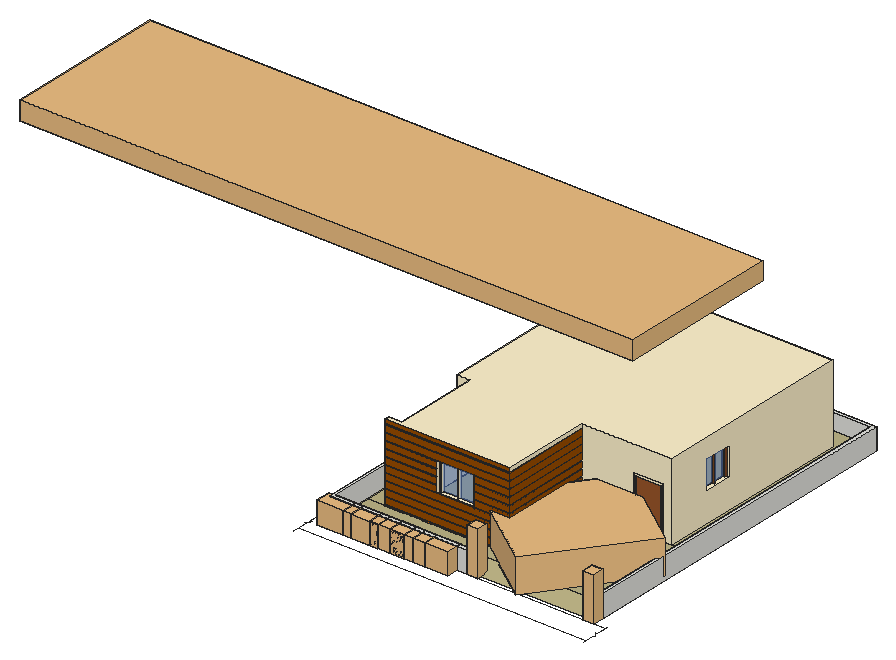
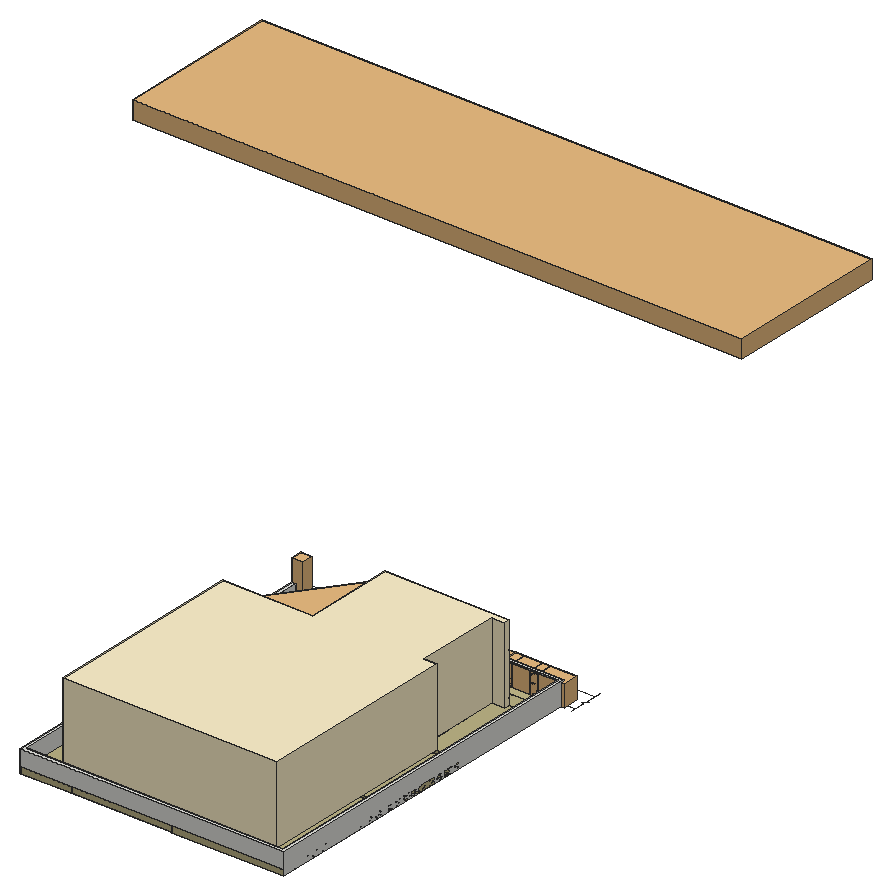
# SketchUp Ruby script. Lengths in inches.
U = 1.inch
M = Sketchup.active_model
def pt(a) = Geom::Point3d.new(a.map { |v| v * U })
def face(e, loops, mat)
  f = e.add_face(loops[0].map { |a| pt(a) })
  loops[1..].each { |l| e.add_face(l.map { |a| pt(a) }).erase! }
  f.material = f.back_material = mat if mat
  f
end
# faces: each face lists its corners as indices into pts; further lists are holes
def faces(e, pts, list, mat = nil) = list.each { |f| face(e, (f[0].is_a?(Array) ? f : [f]).map { |l| l.map { |i| pts[i] } }, mat) }
# xy, xz, yz: faces in a plane at the given z, y or x. An outline is a flat list of corners, or four numbers for a rectangle; further outlines are holes
def ring(l) = l.size == 4 ? [[l[0], l[1]], [l[2], l[1]], [l[2], l[3]], [l[0], l[3]]] : l.each_slice(2).to_a
def flat(e, list, mat, &to3) = list.each { |f| face(e, (f[0].is_a?(Array) ? f : [f]).map { |l| ring(l).map { |u, v| to3.(u, v) } }, mat) }
def xy(e, z, list, mat = nil) = flat(e, list, mat) { |x, y| [x, y, z] }
def xz(e, y, list, mat = nil) = flat(e, list, mat) { |x, z| [x, y, z] }
def yz(e, x, list, mat = nil) = flat(e, list, mat) { |y, z| [x, y, z] }
def lines(e, pts, list) = list.each { |a, b| e.add_line(pt(pts[a]), pt(pts[b])) }
# prism: a flat outline (further loops are holes) pulled along v
def prism(e, loops, v, mat = nil)
  f = face(e, loops, mat); d = Geom::Vector3d.new(v.map { |x| x * U })
  f.pushpull(f.normal.samedirection?(d) ? d.length : -d.length)
end
def box(e, o, s, mat = nil) = prism(e, [[o, [o[0] + s[0], o[1], o[2]], [o[0] + s[0], o[1] + s[1], o[2]], [o[0], o[1] + s[1], o[2]]]], [0, 0, s[2]], mat)
def at(x, y, z, deg = 0) = Geom::Transformation.translation(pt([x, y, z])) * Geom::Transformation.rotation(ORIGIN, Z_AXIS, deg.degrees)
def axes(o, x, y, z) = Geom::Transformation.new([*x, 0, *y, 0, *z, 0, *pt(o).to_a, 1])
def part(name) = M.definitions.add(name)
# library, detail: a bought-in or finely detailed component or shape, given as its bounding box
def library(name, o, s) = part(name).tap { |d| box(d.entities, o, s) }
def detail(e, o, s) = box(e.add_group.entities, o, s)
def put(e, d, t, mat = nil) = e.add_instance(d, t).tap { |i| i.material = mat if mat }
def group(e, t, mat = nil) = e.add_group.tap { |g| g.transformation = t; g.material = mat if mat }.entities
root = M.entities
M.materials.add("[Color C06]").color = [204, 102, 0]
M.materials.add("[Color C07]").color = [153, 76, 0]
M.materials.add("[Color C08]").color = [102, 51, 0]
M.materials.add("[Color D01]").color = [255, 242, 204]
M.materials.add("[Color M06]").color = [86, 86, 86]
M.materials.add("[Tile Ceramic Natural]").color = [189, 180, 134]
M.materials.add("[Translucent Glass Blue]").color = [100, 149, 237]
M.materials["[Translucent Glass Blue]"].alpha = 0.5
M.materials.add("[Wood Cherry Original]").color = [152, 86, 42]
M.materials.add("[Wood Veneer 01]").color = [120, 70, 37]
c1 = library("lvt__Defintion3",[-70.01,-133.44,604.33],[1000,265.15,30.32])
c2 = library("Group\#14",[0,0,0],[56.8,25.91,35.15])
c3 = library("Group\#15",[0,0,0],[56.8,25.91,35.15])
c4 = part("House+plant_11")
put(c4.entities,c1,at(96.28,168.2,0))
put(c4.entities,c2,at(305.6,289.78,0))
put(c4.entities,c2,at(349.27,289.78,0))
put(c4.entities,c3,at(392.14,289.78,0))
put(c4.entities,c2,at(425.32,289.78,0))
put(c4.entities,c2,at(463.51,289.78,0))
c5 = library("Group172\#1",[8097.16,1237.06,0],[18,18,72])
c6 = library("002 Bmw M4 + mat3.4 2017",[-252.8,19.48,9.01],[196.94,171.32,55.15])
c7 = part("new bloSDFck")
p = [[-0.99,-2.25,0],[-22.01,-2.25,0],[-0.99,-4.5,0],[-0.99,0,0],[0.99,0,0],[0.99,-4.5,0],
  [-24,-4.5,0],[-24,0,0],[-22.01,0,0],[-22.01,-4.5,0],[22.01,-4.5,0],[22.01,0,0],
  [24,0,0],[24,-4.5,0],[24,4.5,0],[-24,4.5,0],[22.01,-2.25,0],[0.99,-2.25,0]]
lines(c7.entities,p,[[0,1],[2,3],[4,5],[6,7],[7,8],[8,9],[10,11],[11,12],[12,13],[13,6],[13,14],[6,15],
  [15,14],[12,7],[16,17]])
c8 = part("A$C63CB6BFC")
p = [[-24,-4.5,0],[24,-4.5,0],[24,0,0],[-24,0,0],[22.01,2.25,0],[1.02,2.25,0],
  [-0.96,2.25,0],[-22.01,2.25,0],[-0.96,4.5,0],[-0.96,0,0],[1.02,0,0],[1.02,4.5,0],
  [-22.01,0,0],[-22.01,4.5,0],[22.01,0,0],[24,4.5,0],[-24,4.5,0],[22.01,4.5,0]]
lines(c8.entities,p,[[0,1],[2,3],[4,5],[6,7],[8,9],[9,10],[10,11],[3,12],[12,13],[14,2],[15,16],[15,1],
  [16,0],[17,14]])
c9 = part("A$C1F62275E")
p = [[30,-4.5,0],[-30,-4.5,0],[-30,0,0],[30,0,0],[-28.01,2.25,0],[-0.99,2.25,0],
  [0.99,2.25,0],[28.01,2.25,0],[0.99,4.5,0],[0.99,0,0],[-0.99,0,0],[-0.99,4.5,0],
  [28.01,0,0],[28.01,4.5,0],[-28.01,4.5,0],[-28.01,0,0],[-30,4.5,0],[30,4.5,0]]
lines(c9.entities,p,[[0,1],[2,3],[4,5],[6,7],[8,9],[9,10],[10,11],[3,12],[12,13],[14,15],[15,2],[16,17],
  [16,1],[17,0]])
c10 = part("VEN")
p = [[-4.5,-11.98,0],[4.5,-11.98,0],[2.25,10,0],[2.25,-10,0],[0,-11.98,0],[0,11.98,0],
  [0,-10,0],[4.5,-10,0],[4.5,10,0],[0,10,0],[4.5,11.98,0],[-4.5,11.98,0]]
lines(c10.entities,p,[[0,1],[2,3],[4,5],[6,7],[8,9],[1,10],[0,11],[10,11]])
c11 = part("Group92\#2")
xy(c11.entities,0,[[0,0,25,44]],"[Translucent Glass Blue]")
c12 = part("Group90\#1")
xy(c12.entities,0,[[0,0,0,48,60,48,60,0,56,0,56,44,31,44,31,0,29,0,29,44,4,44,4,0]])
xy(c12.entities,4,[[0,0,4,0,4,44,29,44,29,0,31,0,31,44,56,44,56,0,60,0,60,48,0,48]],"[Color M06]")
xz(c12.entities,0,[[0,0,4,4],[29,0,31,4],[56,0,60,4]])
xz(c12.entities,44,[[4,0,29,4],[31,0,56,4]])
xz(c12.entities,48,[[0,0,60,4]])
yz(c12.entities,0,[[0,0,48,4]])
yz(c12.entities,4,[[0,0,44,4]])
yz(c12.entities,29,[[0,0,44,4]])
yz(c12.entities,31,[[0,0,44,4]])
yz(c12.entities,56,[[0,0,44,4]])
yz(c12.entities,60,[[0,0,48,4]])
p = [[29,0,0],[4,0,0],[56,0,0],[31,0,0],[0.08,0.08,0],[0.08,0.08,4]]
lines(c12.entities,p,[[0,1],[2,3],[4,5]])
put(c12.entities,c11,at(4,0,2))
put(c12.entities,c11,at(31,0,2))
c13 = part("Group103\#2")
xy(c13.entities,0,[[0,0,19,44]],"[Translucent Glass Blue]")
c14 = part("Group101\#1")
prism(c14.entities,[[[25,44,0],[25,0,0],[23,0,0],[23,44,0],[4,44,0],[4,0,0],[0,0,0],[0,48,0],[48,48,0],[48,0,0],[44,0,0],[44,44,0]]],[0,0,4],"[Wood Veneer 01]")
p = [[44,0,0],[25,0,0],[23,0,0],[4,0,0],[0.08,0.08,0],[0.08,0.08,4]]
lines(c14.entities,p,[[0,1],[2,3],[4,5]])
put(c14.entities,c13,at(4,0,2))
put(c14.entities,c13,at(25,0,2))
c15 = part("Group104\#1")
prism(c15.entities,[[[24,42,0],[24,-42,0],[20,-42,0],[20,38,0],[-20,38,0],[-20,-42,0],[-24,-42,0],[-24,42,0]]],[0,0,5.875])
xy(root,10,[[14.3125,35.45,426,35.45,426,208.5,246,208.5,246,60,14.3125,60]],"[Tile Ceramic Natural]")
xz(root,208.5,[[334,10,374,90]],"[Wood Cherry Original]")
p = [[330,208.5,94],[330,208.5,10],[378,208.5,10],[378,208.5,94],[82.3,510.4,0],[82.31,510.39,0],
  [78.09,524.73,0],[78.08,524.73,0],[82.28,510.42,0],[82.29,510.41,0],[82.43,510.33,0],[82.45,510.33,0],
  [78.04,524.72,0],[78.03,524.71,0],[78.02,524.71,0],[78.01,524.7,0],[78,524.69,0],[77.99,524.68,0],
  [78.1,524.73,0],[82.34,510.37,0],[82.35,510.36,0],[82.32,510.38,0],[82.33,510.375,0],[77.98,524.67,0],
  [77.97,524.66,0],[77.96,524.65,0],[77.95,524.64,0],[82.27,510.43,0],[82.26,510.46,0],[82.27,510.44,0],
  [82.4,510.34,0],[82.41,510.34,0],[82.37,510.35,0],[82.38,510.34,0],[82.42,510.33,0],[82.26,510.47,0],
  [78.07,524.73,0],[77.94,524.63,0],[77.9375,524.62,0],[82.36,510.35,0],[78.05,524.72,0],[77.93,524.61,0],
  [77.92,524.58,0],[77.92,524.57,0],[77.92,524.56,0],[77.93,524.6,0],[114.3,524.71,0],[114.29,524.7,0],
  [114.28,524.69,0],[114.39,524.73,0],[114.37,524.73,0],[114.35,524.73,0],[114.33,524.72,0],[114.27,524.68,0],
  [114.4,524.73,0],[114.36,524.73,0],[114.32,524.72,0],[114.31,524.71,0],[114.24,524.65,0],[114.23,524.64,0],
  [114.2,524.55,0],[114.2,524.53,0],[114.21,524.61,0],[114.21,524.6,0],[114.25,524.66,0],[114.2,524.57,0],
  [114.2,524.56,0],[114.26,524.67,0],[114.23,524.63,0],[114.22,524.62,0],[114.21,524.58,0],[55.55,524.73,0],
  [55.54,524.72,0],[55.58,524.73,0],[55.57,524.73,0],[51.83,524.66,0],[51.82,524.67,0],[51.875,524.53,0],
  [51.875,524.55,0],[51.81,524.68,0],[51.83,524.65,0],[51.87,524.58,0],[51.86,524.6,0],[51.8,524.69,0],
  [51.79,524.7,0],[51.85,524.63,0],[51.84,524.64,0],[51.87,524.57,0],[51.85,524.62,0],[51.875,524.56,0],
  [51.86,524.61,0],[102.17,511.09,0],[102.18,511.09,0],[102.12,511.12,0],[102.13,511.11,0],[102.07,511.18,0],
  [102.07,511.17,0],[102.0625,511.19,0],[102.14,511.1,0],[102.15,511.1,0],[102.1,511.14,0],[102.11,511.125,0],
  [102.19,511.08,0],[102.06,511.2,0],[102.08,511.16,0],[102.09,511.15,0]]
lines(root,p,[[0,1],[2,3],[4,5],[6,7],[8,9],[10,11],[12,13],[14,15],[15,16],[16,17],[18,6],[19,20],
  [21,22],[23,24],[25,26],[9,4],[27,8],[22,19],[28,29],[30,31],[32,33],[29,27],[34,10],[35,28],
  [31,34],[7,36],[5,21],[17,23],[24,25],[26,37],[37,38],[39,32],[36,40],[13,14],[20,39],[33,30],
  [40,12],[38,41],[42,43],[43,44],[45,42],[41,45],[46,47],[47,48],[49,50],[51,52],[48,53],[54,49],
  [50,55],[55,51],[52,56],[57,46],[56,57],[58,59],[60,61],[62,63],[64,58],[65,66],[53,67],[67,64],
  [68,69],[63,70],[59,68],[69,62],[70,65],[66,60],[71,72],[73,74],[74,71],[75,76],[77,78],[76,79],
  [80,75],[81,82],[83,84],[85,86],[87,81],[86,80],[88,85],[79,83],[78,89],[82,90],[89,87],[90,88],
  [91,92],[93,94],[95,96],[97,95],[94,98],[99,91],[100,101],[92,102],[101,93],[103,97],[104,105],[96,104],
  [105,100],[98,99]])
put(root,c4,at(-311.65,-308.5,0),"[Color C07]")
g1 = group(root,at(42,60,0),"[Tile Ceramic Natural]")
xy(g1,0,[[-27.6875,-54,-27.6875,148.5,21,148.5,21,100.5,30,100.5,30,157.5,-42,157.5,-42,301.5,9,301.5,9,306,-42,306,-42,516,141,516,141,468,306,468,306,516,389.04,516,389.04,-54],[9,148.5,21,153]])
xy(g1,1,[[141,468,306,477],[141,477,306,516]])
xy(g1,10,[[-27.6875,-24.55,389.04,-24.55,389.04,516,306,516,306,468,141,468,141,516,-42,516,-42,306,9,306,9,301.5,-42,301.5,-42,157.5,30,157.5,30,100.5,21,100.5,21,148.5,-27.6875,148.5],[21,100.5,30,153],[0,148.5,9,157.5],[9,148.5,21,153],[9,153,30,157.5],
  [0,301.5,9,306],[141,477,306,516]])
xz(g1,100.5,[[21,0,30,10]])
xz(g1,148.5,[[-27.6875,0,9,10],[9,0,21,10]])
xz(g1,153,[[9,0,21,10]])
xz(g1,157.5,[[-42,0,30,10],[9,10,30,130]])
xz(g1,301.5,[[-42,0,9,10]])
xz(g1,306,[[-42,0,9,10]])
xz(g1,468,[[141,0,145.5,1],[145.5,0,306,1],[141,1,145.5,10],[145.5,1,306,10]])
xz(g1,477,[[141,1,306,10]])
xz(g1,516,[[-42,0,141,10],[306,0,389.04,10],[141,1,306,10]])
yz(g1,-42,[[157.5,0,301.5,10],[306,0,516,10]])
yz(g1,-27.6875,[[-54,0,-24.55,10,148.5,10,148.5,0]])
yz(g1,9,[[148.5,0,153,10],[301.5,0,306,10],[301.5,10,306,130]])
yz(g1,21,[[100.5,0,148.5,10],[148.5,0,153,10]])
yz(g1,30,[[100.5,0,153,10],[153,0,157.5,10],[153,10,157.5,130]])
yz(g1,141,[[468,0,516,1],[468,1,477,10],[477,1,516,10]])
yz(g1,306,[[468,0,516,1],[468,1,477,10],[477,1,516,10]])
yz(g1,389.04,[[-54,0,516,0,516,10,-24.55,10]])
p = [[389.04,-24.55,10],[384,-24.55,10],[-27.6875,-24.55,10],[-27.6875,-54,0],[389.04,-54,0],[145.5,468,10],
  [145.5,468,130],[204,148.5,10],[384,148.5,10]]
faces(g1,p,[[0,1,2,3,4]])
lines(g1,p,[[5,6],[7,8],[8,1]])
put(root,c5,at(-7683.16,-1237.06,0))
put(root,c5,at(-7872.16,-1237.06,0))
g2 = group(root,at(-21.27,-51.32,0))
xy(g2,0,[[21.27,51.32,21.27,627.32,453.27,627.32,453.27,69.32,447.27,69.32,447.27,621.32,27.27,621.32,27.27,57.32,246.27,57.32,246.27,51.32],[435.27,51.32,453.27,51.32,453.27,65.32,447.27,65.32,447.27,69.32,435.27,69.32],[447.27,65.32,453.27,69.32]])
xy(g2,36,[[21.27,51.32,246.27,51.32,246.27,57.32,27.27,57.32,27.27,621.32,447.27,621.32,447.27,65.32,453.27,65.32,453.27,627.32,21.27,627.32]])
xz(g2,51.32,[[21.27,0,246.27,36]])
xz(g2,57.32,[[27.27,0,246.27,36]])
xz(g2,65.32,[[447.27,0,453.27,36]])
xz(g2,621.32,[[27.27,0,447.27,36]])
xz(g2,627.32,[[21.27,0,453.27,36]])
yz(g2,21.27,[[51.32,0,627.32,36]])
yz(g2,27.27,[[57.32,0,621.32,36]])
yz(g2,246.27,[[51.32,0,57.32,36]])
yz(g2,447.27,[[65.32,0,69.32,36],[69.32,0,621.32,36]])
yz(g2,453.27,[[65.32,0,627.32,36]])
p = [[3.02,34.2,0],[3.02,51.32,0],[246.27,69.32,0],[264.27,69.32,0],[471.91,51.32,0],[453.27,51.32,0],
  [471.91,26.49,0],[474.93,26.49,0],[468.5,34.2,0],[471.91,11.05,0],[3.02,11.05,0],[264.27,51.32,0],
  [435.27,51.32,0],[471.91,34.2,0],[21.27,51.32,0],[3.02,26.49,0],[0,26.49,0],[6.44,34.2,0],
  [3.02,0,0],[471.91,5.47,0],[246.27,51.32,0],[471.91,55.57,0],[3.02,60,0],[246.27,57.32,0]]
lines(g2,p,[[0,1],[2,3],[4,5],[6,7],[7,8],[9,10],[11,12],[13,4],[3,11],[14,1],[8,13],[10,15],
  [15,16],[17,0],[18,10],[19,9],[16,17],[20,11],[4,21],[1,22],[23,2],[9,6]])
put(root,c6,at(130.44,52.04,0,-126.296))
put(root,c7,at(46.5,289.5,10,90))
put(root,c8,axes([144,532.5,10],[1,0,0],[0,-1,0],[0,0,1]))
put(root,c9,at(158,64.5,10))
put(root,c10,at(214.58,532.5,10,-90))
g3 = group(root,at(-18.27,-51.32,10),"[Color D01]")
xy(g3,0,[[396.27,259.82,396.27,268.82,402.27,268.82,402.27,579.32,366.27,579.32,366.27,588.32,411.27,588.32,411.27,259.82],[364.27,579.32,366.27,584.82]])
xy(g3,0,[[60.27,111.32,264.27,113.32],[60.27,113.32,60.27,120.32,81.27,120.32,81.27,211.82,90.27,211.82,90.27,120.32,255.27,120.32,255.27,268.82,348.27,268.82,348.27,259.82,262.27,259.82,262.27,113.32],[262.27,113.32,264.27,259.82]],"[Color C06]")
xy(g3,1.9375,[[262.27,113.32,264.27,259.82]])
xy(g3,1.9375,[[60.27,111.32,262.27,113.32],[262.27,111.32,264.27,113.32]],"[Color C06]")
xy(g3,11.8125,[[60.27,111.32,262.27,113.32],[262.27,111.32,264.27,113.32],[262.27,113.32,264.27,259.82]],"[Color C06]")
xy(g3,13.75,[[60.27,111.32,262.27,113.32],[262.27,111.32,264.27,113.32],[262.27,113.32,264.27,259.82]])
xy(g3,23.625,[[60.27,111.32,262.27,113.32],[262.27,111.32,264.27,113.32],[262.27,113.32,264.27,259.82]],"[Color C06]")
xy(g3,25.5625,[[262.27,113.32,264.27,259.82]])
xy(g3,25.5625,[[60.27,111.32,262.27,113.32],[262.27,111.32,264.27,113.32]],"[Color C06]")
xy(g3,35.4375,[[60.27,111.32,262.27,113.32],[262.27,111.32,264.27,113.32],[262.27,113.32,264.27,259.82]],"[Color C06]")
xy(g3,37.375,[[60.27,111.32,262.27,113.32],[262.27,111.32,264.27,113.32],[262.27,113.32,264.27,259.82]])
xy(g3,47.25,[[262.27,113.32,264.27,259.82]],"[Color C06]")
xy(g3,47.25,[[60.27,111.32,262.27,113.32],[262.27,111.32,264.27,113.32]],"[Color C08]")
xy(g3,48,[[402.27,328.82,411.27,376.82]])
xy(g3,48.08,[[146.35,111.32,206.35,113.32],[146.35,113.32,206.35,120.32]])
xy(g3,49.1875,[[60.27,111.32,146.35,113.32],[262.27,113.32,264.27,259.82]])
xy(g3,49.1875,[[206.35,111.32,262.27,113.32],[262.27,111.32,264.27,113.32]],"[Color C06]")
xy(g3,59.0625,[[60.27,111.32,146.35,113.32]])
xy(g3,59.0625,[[262.27,113.32,264.27,259.82]],"[Color C06]")
xy(g3,59.0625,[[206.35,111.32,262.27,113.32],[262.27,111.32,264.27,113.32]],"[Color C08]")
xy(g3,61,[[60.27,111.32,146.35,113.32],[262.27,113.32,264.27,259.82]])
xy(g3,61,[[206.35,111.32,262.27,113.32],[262.27,111.32,264.27,113.32]],"[Color C06]")
xy(g3,70.875,[[60.27,111.32,146.35,113.32]])
xy(g3,70.875,[[262.27,113.32,264.27,259.82]],"[Color C06]")
xy(g3,70.875,[[206.35,111.32,262.27,113.32],[262.27,111.32,264.27,113.32]],"[Color C08]")
xy(g3,72.8125,[[60.27,111.32,146.35,113.32],[206.35,111.32,262.27,113.32],[262.27,111.32,264.27,113.32],[262.27,113.32,264.27,259.82]])
xy(g3,82.6875,[[60.27,111.32,146.35,113.32]])
xy(g3,82.6875,[[262.27,113.32,264.27,259.82]],"[Color C06]")
xy(g3,82.6875,[[206.35,111.32,262.27,113.32],[262.27,111.32,264.27,113.32]],"[Color C08]")
xy(g3,84,[[348.27,259.82,396.27,268.82]])
xy(g3,84.625,[[60.27,111.32,146.35,113.32],[206.35,111.32,262.27,113.32],[262.27,111.32,264.27,113.32],[262.27,113.32,264.27,259.82]])
xy(g3,94.5,[[60.27,111.32,146.35,113.32]])
xy(g3,94.5,[[262.27,113.32,264.27,259.82]],"[Color C06]")
xy(g3,94.5,[[206.35,111.32,262.27,113.32],[262.27,111.32,264.27,113.32]],"[Color C08]")
xy(g3,96,[[402.27,328.82,411.27,376.82]])
xy(g3,96.08,[[146.35,111.32,206.35,120.32]])
xy(g3,96.4375,[[262.27,113.32,264.27,259.82]])
xy(g3,96.4375,[[60.27,111.32,262.27,113.32],[262.27,111.32,264.27,113.32]],"[Color C06]")
xy(g3,106.3125,[[262.27,113.32,264.27,259.82]],"[Color C06]")
xy(g3,106.3125,[[60.27,111.32,262.27,113.32],[262.27,111.32,264.27,113.32]],"[Color C08]")
xy(g3,108.25,[[60.27,111.32,262.27,113.32],[262.27,111.32,264.27,113.32],[262.27,113.32,264.27,259.82]])
xy(g3,118.125,[[262.27,113.32,264.27,259.82]],"[Color C06]")
xy(g3,118.125,[[60.27,111.32,262.27,113.32],[262.27,111.32,264.27,113.32]],"[Color C08]")
xy(g3,120.0625,[[262.27,113.32,264.27,259.82]],"[Color C06]")
xy(g3,120.0625,[[60.27,111.32,262.27,113.32],[262.27,111.32,264.27,113.32]],"[Color C08]")
xy(g3,126,[[60.27,111.32,264.27,111.32,264.27,259.82,411.27,259.82,411.27,588.32,60.27,588.32,60.27,259.82,81.27,259.82,81.27,120.32,60.27,120.32]])
xz(g3,111.32,[[60.27,1.9375,264.27,11.8125],[60.27,13.75,264.27,23.625],[60.27,25.5625,264.27,35.4375],[60.27,37.375,264.27,47.25],[60.27,49.1875,146.35,59.0625],
  [206.35,49.1875,264.27,59.0625],[60.27,61,146.35,70.875],[206.35,61,264.27,70.875],[60.27,72.8125,146.35,82.6875],[206.35,72.8125,264.27,82.6875],
  [60.27,84.625,146.35,94.5],[206.35,84.625,264.27,94.5],[60.27,96.4375,264.27,106.3125],[60.27,108.25,264.27,118.125],[60.27,120.0625,264.27,126]],"[Color C07]")
xz(g3,113.32,[[60.27,0,262.27,1.9375],[262.27,0,264.27,1.9375],[60.27,11.8125,262.27,13.75],[262.27,11.8125,264.27,13.75],[60.27,23.625,262.27,25.5625],
  [262.27,23.625,264.27,25.5625],[60.27,35.4375,262.27,37.375],[262.27,35.4375,264.27,37.375],[60.27,47.25,262.27,47.25,262.27,49.1875,206.35,49.1875,206.35,48.08,146.35,48.08,146.35,49.1875,60.27,49.1875],[262.27,47.25,264.27,49.1875],
  [60.27,59.0625,146.35,61],[206.35,59.0625,262.27,61],[262.27,59.0625,264.27,61],[60.27,70.875,146.35,72.8125],[206.35,70.875,262.27,72.8125],
  [262.27,70.875,264.27,72.8125],[60.27,82.6875,146.35,84.625],[206.35,82.6875,262.27,84.625],[262.27,82.6875,264.27,84.625],[262.27,94.5,264.27,96.4375],
  [60.27,106.3125,262.27,108.25],[262.27,106.3125,264.27,108.25]],"[Color C06]")
xz(g3,113.32,[[60.27,118.125,262.27,120.0625],[262.27,118.125,264.27,120.0625]],"[Color C08]")
xz(g3,120.32,[[60.27,0,81.27,126],[[90.27,0,255.27,120],[146.35,48.08,206.35,96.08]]])
xz(g3,259.82,[[60.27,0,81.27,126]])
xz(g3,259.82,[[264.27,0,348.27,0,348.27,84,396.27,84,396.27,0,411.27,0,411.27,126,264.27,126]],"[Color D01]")
xz(g3,268.82,[[255.27,0,255.27,120,402.27,120,402.27,0,396.27,0,396.27,84,348.27,84,348.27,0]])
xz(g3,328.82,[[402.27,48,411.27,96]])
xz(g3,376.82,[[402.27,48,411.27,96]])
xz(g3,579.32,[[69.27,0,201.27,120],[205.77,0,259.77,120],[264.27,0,402.27,120]],"[Color D01]")
xz(g3,588.32,[[60.27,0,411.27,126]],"[Color D01]")
yz(g3,60.27,[[111.32,0,113.32,1.9375],[113.32,0,113.32,1.9375,111.32,1.9375,111.32,11.8125,113.32,11.8125,113.32,13.75,111.32,13.75,111.32,23.625,113.32,23.625,113.32,25.5625,111.32,25.5625,111.32,35.4375,113.32,35.4375,113.32,37.375,111.32,37.375,111.32,47.25,113.32,47.25,113.32,49.1875,111.32,49.1875,111.32,59.0625,113.32,59.0625,113.32,61,111.32,61,111.32,70.875,113.32,70.875,113.32,72.8125,111.32,72.8125,111.32,82.6875,113.32,82.6875,113.32,84.625,111.32,84.625,111.32,94.5,113.32,94.5,113.32,96.4375,111.32,96.4375,111.32,106.3125,113.32,106.3125,113.32,108.25,111.32,108.25,111.32,118.125,113.32,118.125,113.32,120.0625,111.32,120.0625,111.32,126,120.32,126,120.32,0],[259.82,0,588.32,126],[111.32,11.8125,113.32,13.75],[111.32,23.625,113.32,25.5625],
  [111.32,35.4375,113.32,37.375],[111.32,47.25,113.32,49.1875],[111.32,59.0625,113.32,61],[111.32,70.875,113.32,72.8125],[111.32,82.6875,113.32,84.625],
  [111.32,94.5,113.32,96.4375],[111.32,106.3125,113.32,108.25],[111.32,118.125,113.32,120.0625]])
yz(g3,69.27,[[268.82,0,412.82,120],[417.32,0,579.32,120]])
yz(g3,81.27,[[120.32,0,259.82,126]])
yz(g3,90.27,[[120.32,0,264.32,120]])
yz(g3,146.35,[[111.32,48.08,113.32,49.1875],[113.32,48.08,120.32,48.08,120.32,96.08,113.32,96.08,113.32,94.5,111.32,94.5,111.32,84.625,113.32,84.625,113.32,82.6875,111.32,82.6875,111.32,72.8125,113.32,72.8125,113.32,70.875,111.32,70.875,111.32,61,113.32,61,113.32,59.0625,111.32,59.0625,111.32,49.1875,113.32,49.1875],[111.32,59.0625,113.32,61],[111.32,70.875,113.32,72.8125],[111.32,82.6875,113.32,84.625],
  [111.32,94.5,113.32,96.08]])
yz(g3,206.35,[[111.32,48.08,113.32,49.1875],[113.32,48.08,113.32,49.1875,111.32,49.1875,111.32,59.0625,113.32,59.0625,113.32,61,111.32,61,111.32,70.875,113.32,70.875,113.32,72.8125,111.32,72.8125,111.32,82.6875,113.32,82.6875,113.32,84.625,111.32,84.625,111.32,94.5,113.32,94.5,113.32,96.08,120.32,96.08,120.32,48.08],[111.32,59.0625,113.32,61],[111.32,70.875,113.32,72.8125],[111.32,82.6875,113.32,84.625],
  [111.32,94.5,113.32,96.08]])
yz(g3,255.27,[[120.32,0,268.82,120]])
yz(g3,262.27,[[113.32,0,259.82,1.9375],[113.32,11.8125,259.82,13.75],[113.32,23.625,259.82,25.5625],[113.32,35.4375,259.82,37.375],[113.32,47.25,259.82,49.1875],
  [113.32,59.0625,259.82,61],[113.32,70.875,259.82,72.8125],[113.32,82.6875,259.82,84.625],[113.32,94.5,259.82,96.4375],[113.32,106.3125,259.82,108.25],
  [113.32,118.125,259.82,120.0625]],"[Color C06]")
yz(g3,264.27,[[111.32,120.0625,259.82,126]])
yz(g3,264.27,[[111.32,0,113.32,1.9375],[111.32,11.8125,113.32,13.75],[111.32,23.625,113.32,25.5625],[111.32,35.4375,113.32,37.375],[111.32,47.25,113.32,49.1875],
  [111.32,59.0625,113.32,61],[111.32,70.875,113.32,72.8125],[111.32,82.6875,113.32,84.625],[111.32,94.5,113.32,96.4375],[111.32,106.3125,113.32,108.25],
  [111.32,118.125,113.32,120.0625]],"[Color C06]")
yz(g3,264.27,[[111.32,1.9375,259.82,11.8125],[111.32,13.75,259.82,23.625],[111.32,25.5625,259.82,35.4375],[111.32,37.375,259.82,47.25],[111.32,49.1875,259.82,59.0625],
  [111.32,61,259.82,70.875],[111.32,72.8125,259.82,82.6875],[111.32,84.625,259.82,94.5],[111.32,96.4375,259.82,106.3125],[111.32,108.25,259.82,118.125]],"[Color C07]")
yz(g3,348.27,[[259.82,0,268.82,84]])
yz(g3,396.27,[[259.82,0,268.82,84]])
yz(g3,402.27,[[[268.82,0,579.32,120],[328.82,48,376.82,96]]])
yz(g3,411.27,[[[259.82,0,588.32,126],[328.82,48,376.82,96]]],"[Color D01]")
p = [[198.89,111.32,120],[198.89,120.32,120],[352.27,259.82,0],[392.27,259.82,0],[348.27,259.82,0],[352.27,259.82,80],
  [392.27,259.82,80],[396.27,259.82,0]]
lines(g3,p,[[0,1],[2,3],[4,2],[2,5],[5,6],[6,3],[3,7]])
put(g3,c12,axes([146.35,120.32,48.08],[1,0,0],[0,0,1],[0,-1,0]),"[Color D01]")
put(g3,c14,axes([402.27,328.82,48],[0,1,0],[0,0,1],[1,0,0]))
put(g3,c15,axes([372.27,265.69,42],[1,0,0],[0,0,1],[0,-1,0]))
